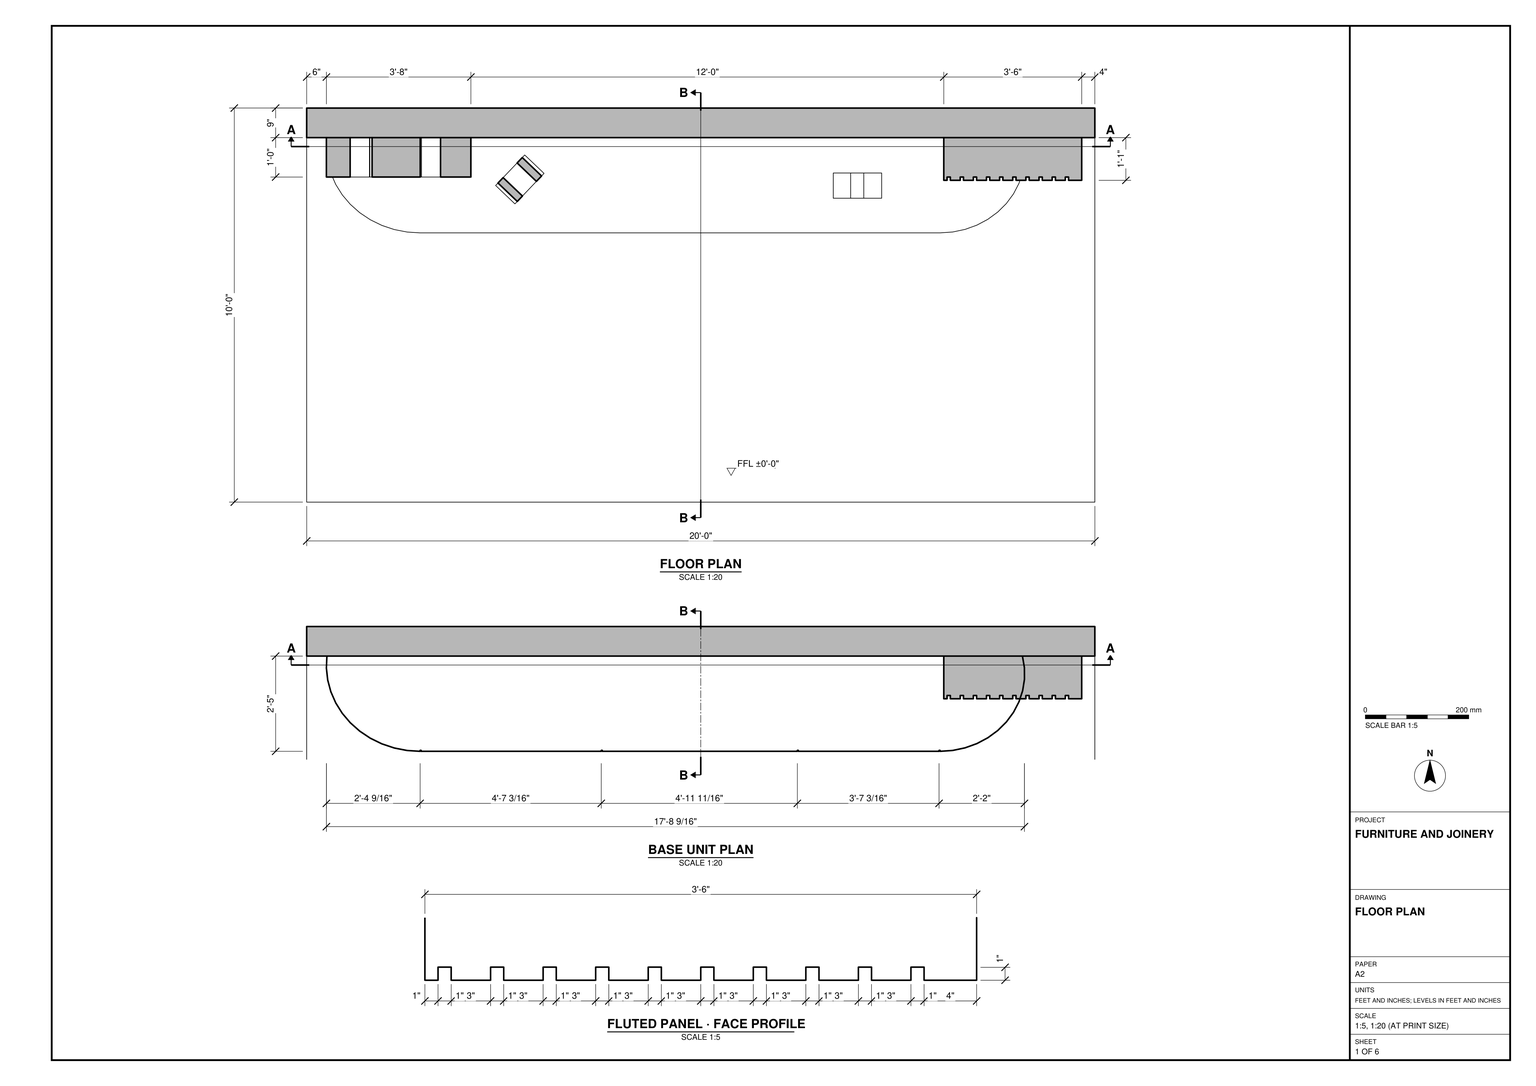
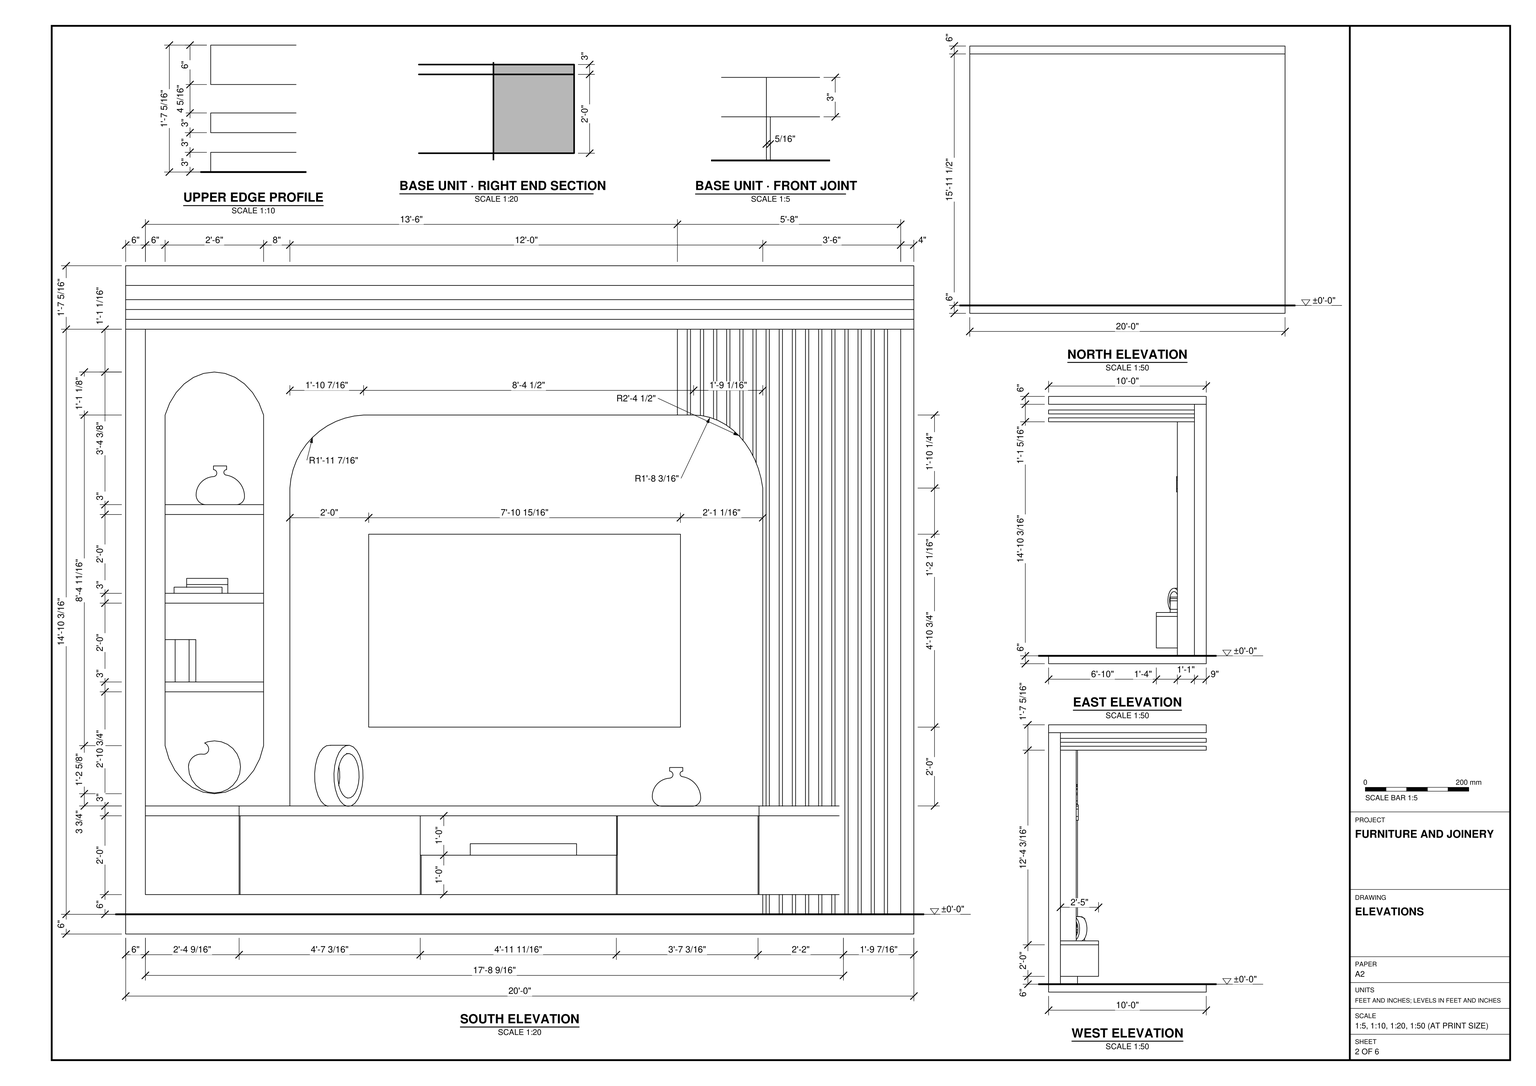
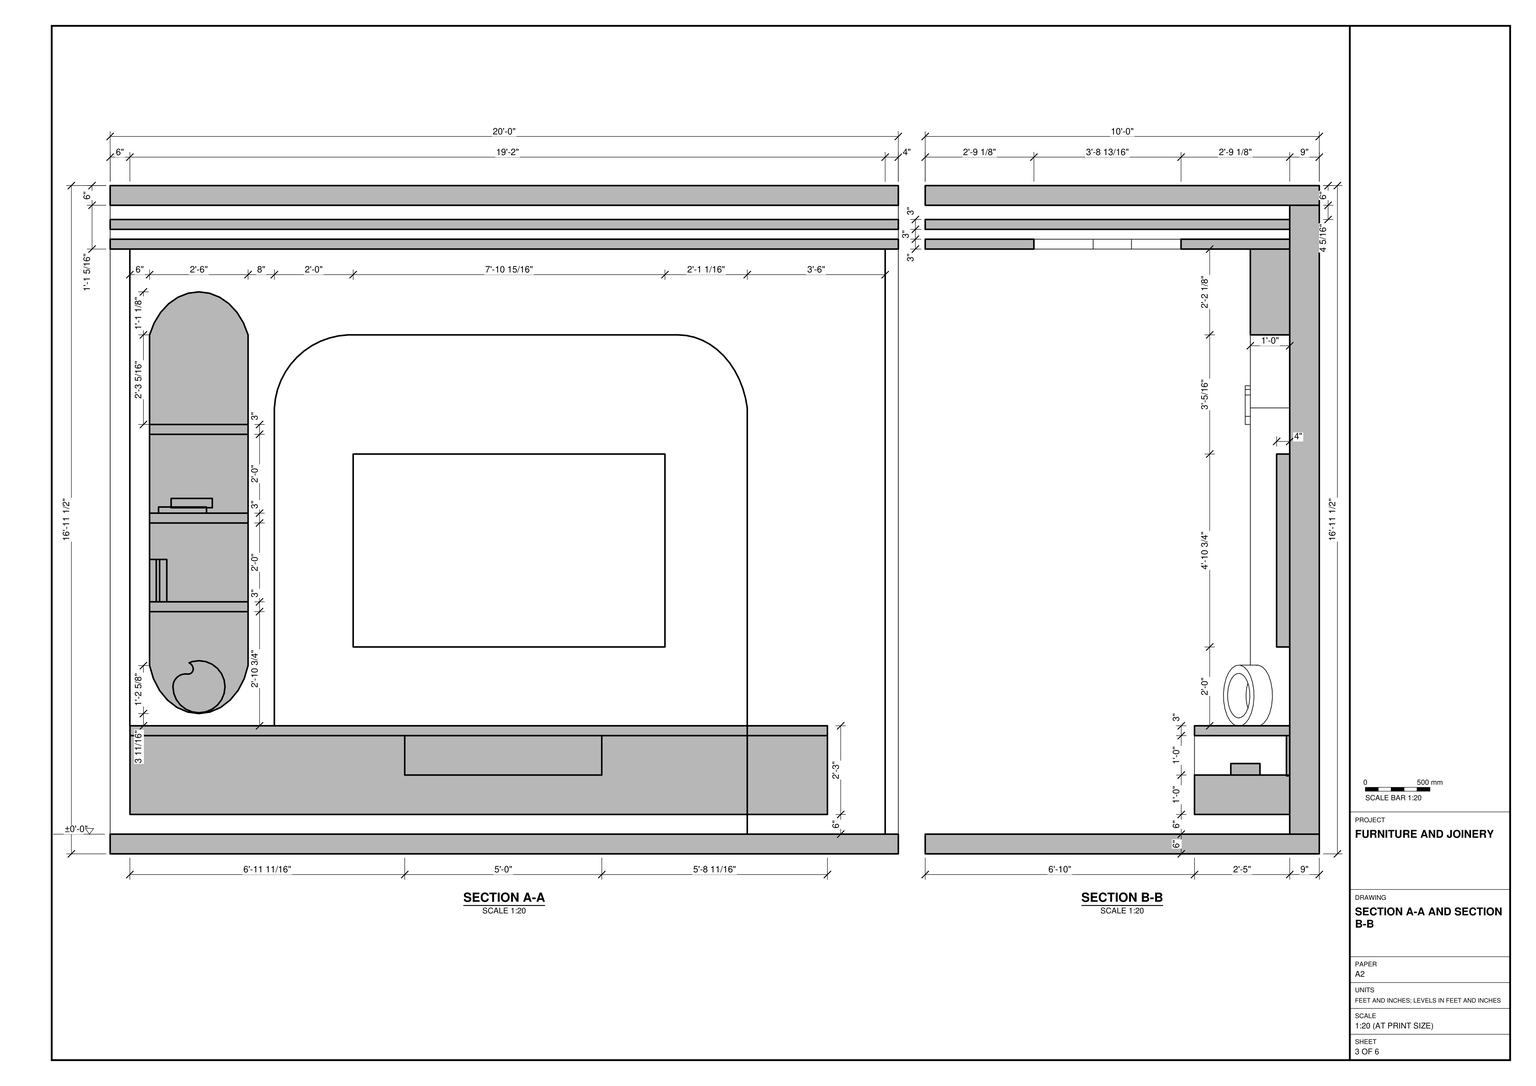
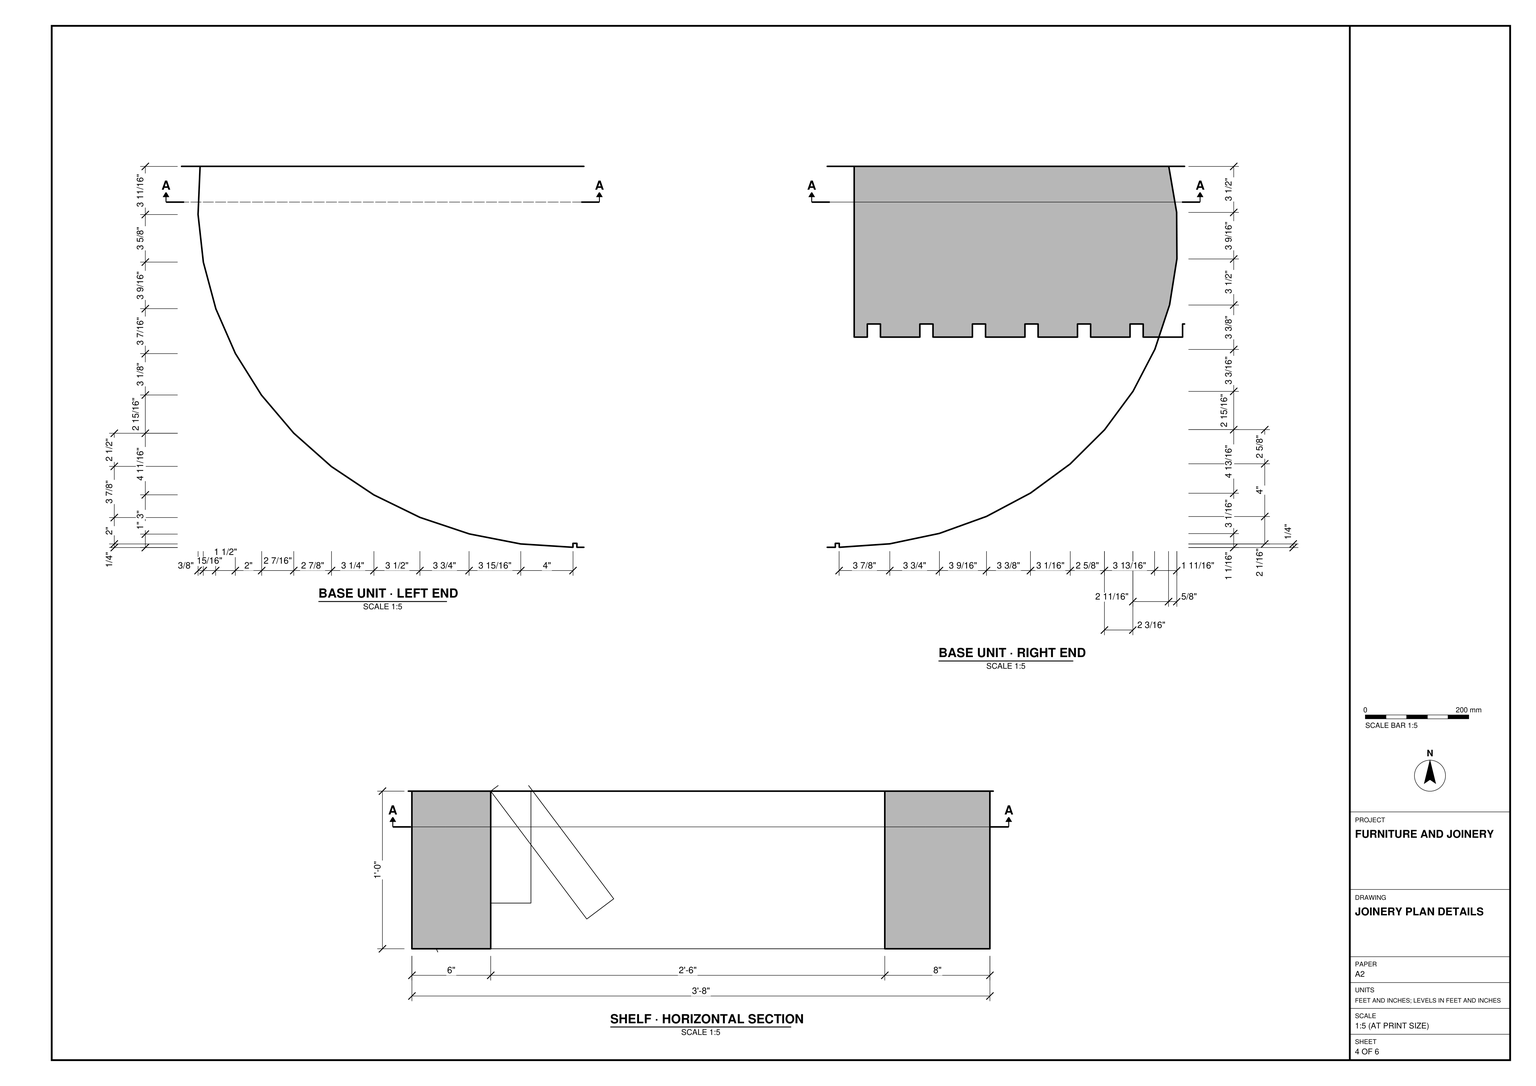
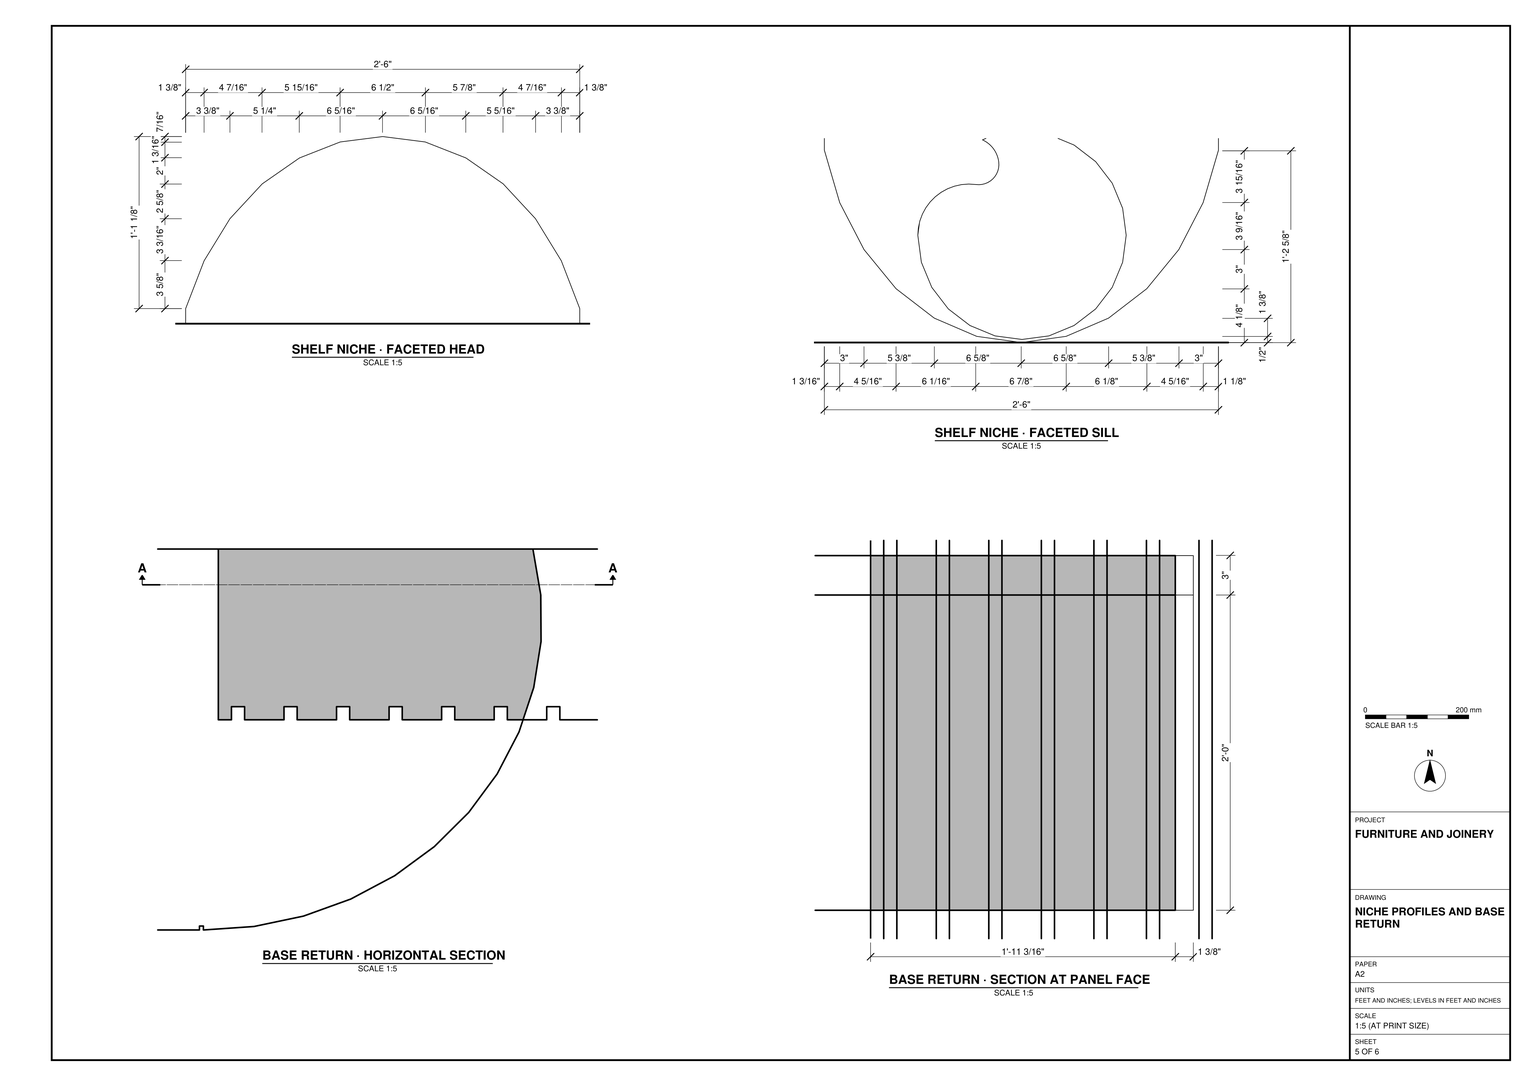
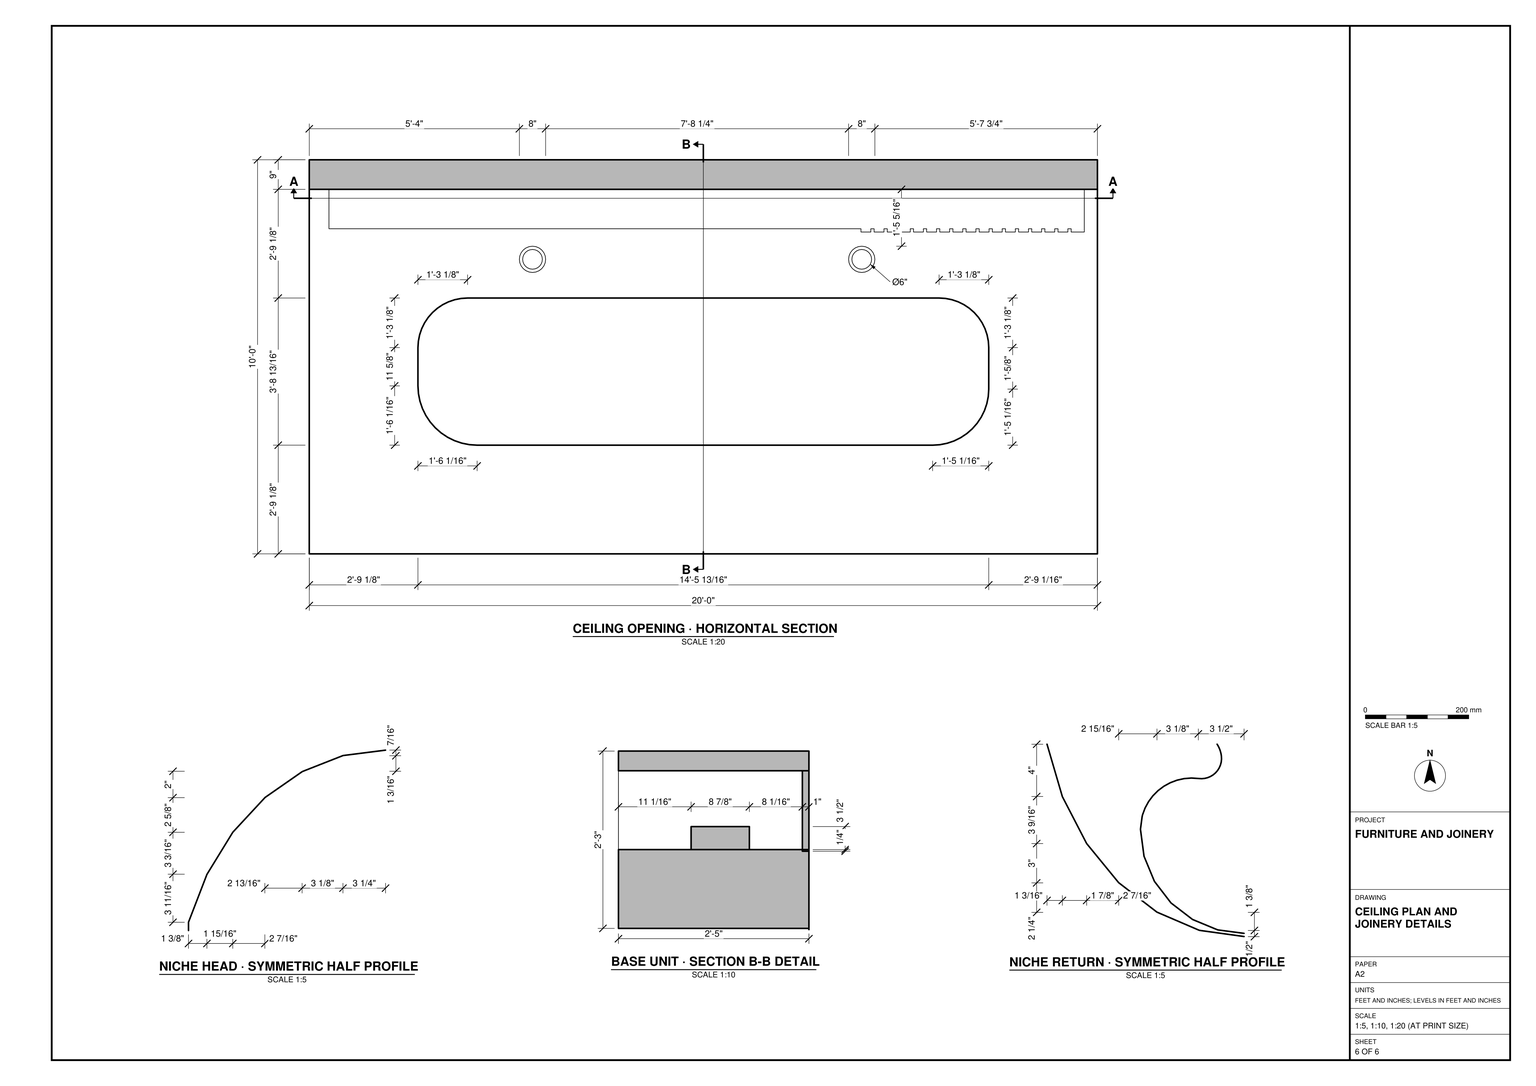
Build the TV wall and its surrounding floor, backing wall and overhead assembly in SketchUp from task_files/diagram_01.pdf. Work in feet and inches. The overall model is 20'-0" wide, 10'-0" deep and 16'-11 1/2" high. Set the finished floor at ±0'-0". Place the 9" backing wall along the north edge of the floor slab and use the south elevation to lay out the joinery.

Run the floating base cabinet beneath the shelving and TV. Follow the base unit plan for the straight front and curved ends, and the sections for the top thickness, divided fronts and open central compartment. Above the cabinet, form a tall, narrow display niche on the left with rounded upper and lower ends and horizontal shelves. Mount the rectangular TV within the wider central recess, keeping the straight head and rounded upper corners of the recess distinct from the TV itself. Model the vertical grooves in the right-hand panel and the stepped horizontal bands beneath the top slab.

Decor and loose items on the shelves and cabinet top may be any suitable library components placed as shown. Keep the shell elements and each joinery or furniture piece in separate groups or components, and use components for repeated parts. Save one SketchUp model as output_files/tv_wall_with_display_shelves_and_floating_storage.skp.

# SketchUp Ruby script. Lengths in inches.
U = 1.inch
M = Sketchup.active_model
def pt(a) = Geom::Point3d.new(a.map { |v| v * U })
def face(e, loops, mat)
  f = e.add_face(loops[0].map { |a| pt(a) })
  loops[1..].each { |l| e.add_face(l.map { |a| pt(a) }).erase! }
  f.material = f.back_material = mat if mat
  f
end
# faces: each face lists its corners as indices into pts; further lists are holes
def faces(e, pts, list, mat = nil) = list.each { |f| face(e, (f[0].is_a?(Array) ? f : [f]).map { |l| l.map { |i| pts[i] } }, mat) }
# xy, xz, yz: faces in a plane at the given z, y or x. An outline is a flat list of corners, or four numbers for a rectangle; further outlines are holes
def ring(l) = l.size == 4 ? [[l[0], l[1]], [l[2], l[1]], [l[2], l[3]], [l[0], l[3]]] : l.each_slice(2).to_a
def flat(e, list, mat, &to3) = list.each { |f| face(e, (f[0].is_a?(Array) ? f : [f]).map { |l| ring(l).map { |u, v| to3.(u, v) } }, mat) }
def xy(e, z, list, mat = nil) = flat(e, list, mat) { |x, y| [x, y, z] }
def xz(e, y, list, mat = nil) = flat(e, list, mat) { |x, z| [x, y, z] }
def yz(e, x, list, mat = nil) = flat(e, list, mat) { |y, z| [x, y, z] }
def lines(e, pts, list) = list.each { |a, b| e.add_line(pt(pts[a]), pt(pts[b])) }
# prism: a flat outline (further loops are holes) pulled along v
def prism(e, loops, v, mat = nil)
  f = face(e, loops, mat); d = Geom::Vector3d.new(v.map { |x| x * U })
  f.pushpull(f.normal.samedirection?(d) ? d.length : -d.length)
end
def box(e, o, s, mat = nil) = prism(e, [[o, [o[0] + s[0], o[1], o[2]], [o[0] + s[0], o[1] + s[1], o[2]], [o[0], o[1] + s[1], o[2]]]], [0, 0, s[2]], mat)
def at(x, y, z, deg = 0) = Geom::Transformation.translation(pt([x, y, z])) * Geom::Transformation.rotation(ORIGIN, Z_AXIS, deg.degrees)
def axes(o, x, y, z) = Geom::Transformation.new([*x, 0, *y, 0, *z, 0, *pt(o).to_a, 1])
def part(name) = M.definitions.add(name)
# library, detail: a bought-in or finely detailed component or shape, given as its bounding box
def library(name, o, s) = part(name).tap { |d| box(d.entities, o, s) }
def detail(e, o, s) = box(e.add_group.entities, o, s)
def put(e, d, t, mat = nil) = e.add_instance(d, t).tap { |i| i.material = mat if mat }
def group(e, t, mat = nil) = e.add_group.tap { |g| g.transformation = t; g.material = mat if mat }.entities
root = M.entities
M.materials.add("[Color A07]").color = [153, 0, 0]
M.materials.add("[Color E05]").color = [255, 255, 0]
M.materials.add("[Color E08]").color = [102, 102, 0]
M.materials.add("[Color L16]").color = [102, 0, 51]
M.materials.add("[Color M00]").color = [255, 255, 255]
M.materials.add("[Color M05]").color = [114, 114, 114]
M.materials.add("[Color M06]").color = [86, 86, 86]
M.materials.add("[Color M07]").color = [58, 58, 58]
M.materials.add("[Color M08]").color = [30, 30, 30]
M.materials.add("[Color M09]").color = [0, 0, 0]
c1 = part("Group\#17")
detail(c1.entities,[0,0,0],[14.74,7.6875,11.79])
g1 = group(root,at(0,0,0))
box(g1,[0,0,0],[240,120,6])
g2 = group(root,at(0,111,6),"[Color M00]")
box(g2,[0,0,0],[240,9,191.5])
g3 = group(root,at(6,99,39),"[Color M00]")
xy(g3,-33,[[188,-1,188,12,230,12,230,-1,226,-1,226,0,225,0,225,-1,222,-1,222,0,221,0,221,-1,218,-1,218,0,217,0,217,-1,214,-1,214,0,213,0,213,-1,210,-1,210,0,209,0,209,-1,206,-1,206,0,205,0,205,-1,202,-1,202,0,201,0,201,-1,198,-1,198,0,197,0,197,-1,194,-1,194,0,193,0,193,-1,190,-1,190,0,189,0,189,-1]])
xy(g3,0,[[0,0,44,12]])
xy(g3,119.04,[[162,-1,162,0,66.45,0,66.45,12,166.95,12,166.95,-1,166,-1,166,0,165,0,165,-1]])
xy(g3,145.17,[[162,-1,165,-1,165,0,166,0,166,-1,169,-1,169,0,170,0,170,-1,173,-1,173,0,174,0,174,-1,177,-1,177,0,178,0,178,-1,181,-1,181,0,182,0,182,-1,185,-1,185,0,186,0,186,-1,189,-1,189,0,190,0,190,-1,193,-1,193,0,194,0,194,-1,197,-1,197,0,198,0,198,-1,201,-1,201,0,202,0,202,-1,205,-1,205,0,206,0,206,-1,209,-1,209,0,210,0,210,-1,213,-1,213,0,214,0,214,-1,217,-1,217,0,218,0,218,-1,221,-1,221,0,222,0,222,-1,225,-1,225,0,226,0,226,-1,230,-1,230,12,0,12,0,0,162,0]])
xz(g3,-1,[[188,-33,189,-33,189,145.17,186,145.17,186,104.375,186.63,102.77,187.46,99.83,188,96.8],[190,-33,193,145.17],[194,-33,197,145.17],[198,-33,201,145.17],[202,-33,205,145.17],
  [206,-33,209,145.17],[210,-33,213,145.17],[214,-33,217,145.17],[218,-33,221,145.17],[222,-33,225,145.17],
  [226,-33,230,145.17],[185,106.59,185,145.17,182,145.17,182,111.27,182.59,110.57,184.18,108.17],[181,112.46,181,145.17,178,145.17,178,115.16,178.78,114.6,180.78,112.73],[177,115.89,177,145.17,174,145.17,174,117.53,174.32,117.41,176.61,116.17],[173,117.91,173,145.17,170,145.17,170,118.74,171.92,118.3125],
  [169,118.89,169,145.17,166,145.17,166,119.04,166.95,119.04],[162,119.04,165,145.17]],"[Color M08]")
xz(g3,0,[[[0,0,44,0,44,96.8,44.32,99.67,45,102.47,46.01,105.18,47.35,107.74,48.99,110.11,50.92,112.27,53.09,114.17,55.48,115.79,58.05,117.1,60.76,118.09,63.58,118.74,66.45,119.04,162,119.04,162,145.17,0,145.17],[21,3.73,17.6,4.2,14.36,5.59,11.46,7.83,9.02,10.81,7.17,14.38,6,18.37,6,119.04,7.4,122.68,9.37,125.89,11.83,128.53,14.66,130.51,17.76,131.73,21,132.14,24.24,131.73,27.34,130.51,30.17,128.53,32.63,125.89,34.6,122.68,36,119.04,36,18.37,34.83,14.38,32.98,10.81,30.54,7.83,27.64,5.59,24.4,4.2]]])
xz(g3,0,[[189,-33,190,145.17],[193,-33,194,145.17],[197,-33,198,145.17],[201,-33,202,145.17],[205,-33,206,145.17],
  [209,-33,210,145.17],[213,-33,214,145.17],[217,-33,218,145.17],[221,-33,222,145.17],[225,-33,226,145.17],
  [186,104.375,186,145.17,185,145.17,185,106.59,185.53,105.56],[182,111.27,182,145.17,181,145.17,181,112.46],[178,115.16,178,145.17,177,145.17,177,115.89],[174,117.53,174,145.17,173,145.17,173,117.91],[170,118.74,170,145.17,169,145.17,169,118.89,169.45,118.86],
  [165,119.04,166,145.17]],"[Color M08]")
xz(g3,12,[[[188,-33,188,96.8,187.46,99.83,186.63,102.77,185.53,105.56,184.18,108.17,182.59,110.57,180.78,112.73,178.78,114.6,176.61,116.17,174.32,117.41,171.92,118.3125,169.45,118.86,166.95,119.04,66.45,119.04,63.58,118.74,60.76,118.09,58.05,117.1,55.48,115.79,53.09,114.17,50.92,112.27,48.99,110.11,47.35,107.74,46.01,105.18,45,102.47,44.32,99.67,44,96.8,44,0,0,0,0,145.17,230,145.17,230,-33],[21,3.73,24.4,4.2,27.64,5.59,30.54,7.83,32.98,10.81,34.83,14.38,36,18.37,36,119.04,34.6,122.68,32.63,125.89,30.17,128.53,27.34,130.51,24.24,131.73,21,132.14,17.76,131.73,14.66,130.51,11.83,128.53,9.37,125.89,7.4,122.68,6,119.04,6,18.37,7.17,14.38,9.02,10.81,11.46,7.83,14.36,5.59,17.6,4.2]]])
yz(g3,0,[[0,0,12,145.17]])
yz(g3,6,[[0,18.37,12,119.04]])
yz(g3,36,[[0,18.37,12,119.04]])
yz(g3,44,[[0,0,12,96.8]])
yz(g3,162,[[-1,119.04,0,145.17]])
yz(g3,165,[[-1,119.04,0,145.17]])
yz(g3,166,[[-1,119.04,0,145.17]])
yz(g3,169,[[-1,118.89,0,145.17]])
yz(g3,170,[[-1,118.74,0,145.17]])
yz(g3,173,[[-1,117.91,0,145.17]])
yz(g3,174,[[-1,117.53,0,145.17]])
yz(g3,177,[[-1,115.89,0,145.17]])
yz(g3,178,[[-1,115.16,0,145.17]])
yz(g3,181,[[-1,112.46,0,145.17]])
yz(g3,182,[[-1,111.27,0,145.17]])
yz(g3,185,[[-1,106.59,0,145.17]])
yz(g3,186,[[-1,104.375,0,145.17]])
yz(g3,188,[[-1,-33,12,96.8]])
yz(g3,189,[[-1,-33,0,145.17]])
yz(g3,190,[[-1,-33,0,145.17]])
yz(g3,193,[[-1,-33,0,145.17]])
yz(g3,194,[[-1,-33,0,145.17]])
yz(g3,197,[[-1,-33,0,145.17]])
yz(g3,198,[[-1,-33,0,145.17]])
yz(g3,201,[[-1,-33,0,145.17]])
yz(g3,202,[[-1,-33,0,145.17]])
yz(g3,205,[[-1,-33,0,145.17]])
yz(g3,206,[[-1,-33,0,145.17]])
yz(g3,209,[[-1,-33,0,145.17]])
yz(g3,210,[[-1,-33,0,145.17]])
yz(g3,213,[[-1,-33,0,145.17]])
yz(g3,214,[[-1,-33,0,145.17]])
yz(g3,217,[[-1,-33,0,145.17]])
yz(g3,218,[[-1,-33,0,145.17]])
yz(g3,221,[[-1,-33,0,145.17]])
yz(g3,222,[[-1,-33,0,145.17]])
yz(g3,225,[[-1,-33,0,145.17]])
yz(g3,226,[[-1,-33,0,145.17]])
yz(g3,230,[[-1,-33,12,145.17]])
p = [[21,12,3.73],[17.6,12,4.2],[17.6,0,4.2],[21,0,3.73],[24.4,12,4.2],[24.4,0,4.2],
  [14.36,12,5.59],[14.36,0,5.59],[27.64,12,5.59],[27.64,0,5.59],[11.46,12,7.83],[11.46,0,7.83],
  [30.54,12,7.83],[30.54,0,7.83],[9.02,12,10.81],[9.02,0,10.81],[32.98,12,10.81],[32.98,0,10.81],
  [7.17,12,14.38],[7.17,0,14.38],[34.83,12,14.38],[34.83,0,14.38],[6,12,18.37],[6,0,18.37],
  [36,12,18.37],[36,0,18.37],[187.46,12,99.83],[188,12,96.8],[188,-1,96.8],[187.46,-1,99.83],
  [44.32,0,99.67],[44,0,96.8],[44,12,96.8],[44.32,12,99.67],[45,0,102.47],[45,12,102.47],
  [186.63,12,102.77],[186.63,-1,102.77],[46.01,0,105.18],[46.01,12,105.18],[185.53,12,105.56],[186,-1,104.375],
  [186,0,104.375],[185.53,0,105.56],[47.35,0,107.74],[47.35,12,107.74],[184.18,12,108.17],[185,0,106.59],
  [185,-1,106.59],[184.18,-1,108.17],[48.99,0,110.11],[48.99,12,110.11],[182.59,12,110.57],[182.59,-1,110.57],
  [50.92,0,112.27],[50.92,12,112.27],[180.78,12,112.73],[182,-1,111.27],[182,0,111.27],[181,0,112.46],
  [181,-1,112.46],[180.78,-1,112.73],[53.09,0,114.17],[53.09,12,114.17],[178.78,12,114.6],[178.78,-1,114.6],
  [55.48,0,115.79],[55.48,12,115.79],[176.61,12,116.17],[178,-1,115.16],[178,0,115.16],[177,0,115.89],
  [177,-1,115.89],[176.61,-1,116.17],[58.05,0,117.1],[58.05,12,117.1],[174.32,12,117.41],[174.32,-1,117.41],
  [60.76,0,118.09],[60.76,12,118.09],[171.92,12,118.3125],[174,-1,117.53],[174,0,117.53],[173,0,117.91],
  [173,-1,117.91],[171.92,-1,118.3125],[63.58,0,118.74],[63.58,12,118.74],[169.45,12,118.86],[170,-1,118.74],
  [170,0,118.74],[169.45,0,118.86],[66.45,0,119.04],[66.45,12,119.04],[166.95,12,119.04],[169,0,118.89],
  [169,-1,118.89],[166.95,-1,119.04],[6,12,119.04],[7.4,12,122.68],[7.4,0,122.68],[6,0,119.04],
  [34.6,12,122.68],[36,12,119.04],[36,0,119.04],[34.6,0,122.68],[9.37,12,125.89],[9.37,0,125.89],
  [32.63,12,125.89],[32.63,0,125.89],[11.83,12,128.53],[11.83,0,128.53],[30.17,12,128.53],[30.17,0,128.53],
  [14.66,12,130.51],[14.66,0,130.51],[27.34,12,130.51],[27.34,0,130.51],[17.76,12,131.73],[17.76,0,131.73],
  [24.24,12,131.73],[24.24,0,131.73],[21,12,132.14],[21,0,132.14]]
faces(g3,p,[[0,1,2,3],[4,0,3,5],[1,6,7,2],[8,4,5,9],[6,10,11,7],[12,8,9,13],[10,14,15,11],[16,12,13,17],
  [14,18,19,15],[20,16,17,21],[18,22,23,19],[24,20,21,25],[26,27,28,29],[30,31,32,33],[34,30,33,35],[36,26,29,37],
  [38,34,35,39],[40,36,37,41,42,43],[44,38,39,45],[46,40,43,47,48,49],[50,44,45,51],[52,46,49,53],[54,50,51,55],[56,52,53,57,58,59,60,61],
  [62,54,55,63],[64,56,61,65],[66,62,63,67],[68,64,65,69,70,71,72,73],[74,66,67,75],[76,68,73,77],[78,74,75,79],[80,76,77,81,82,83,84,85],
  [86,78,79,87],[88,80,85,89,90,91],[92,86,87,93],[94,88,91,95,96,97],[98,99,100,101],[102,103,104,105],[99,106,107,100],[108,102,105,109],
  [106,110,111,107],[112,108,109,113],[110,114,115,111],[116,112,113,117],[114,118,119,115],[120,116,117,121],[118,122,123,119],[122,120,121,123]])
g4 = group(root,at(6,82,36),"[Color M08]")
prism(g4,[[[0.16,29,0],[211.95,29,0],[212.55,25.5,0],[212.57,21.96,0],[212.01,18.46,0],[210.89,15.07,0],[209.23,11.875,0],[207.06,8.94,0],[204.4375,6.34,0],[201.42,4.13,0],[198.08,2.35,0],[194.48,1.06,0],[190.72,0.27,0],[186.86,0,0],[28.54,0,0],[24.56,0.26,0],[20.65,1.02,0],[16.9,2.27,0],[13.375,3.99,0],[10.15,6.15,0],[7.28,8.7,0],[4.83,11.58,0],[2.84,14.76,0],[1.36,18.15,0],[0.4,21.7,0],[0,25.34,0]]],[0,0,3])
g5 = group(root,at(6,82,12),"[Color M00]")
xy(g5,0,[[28.54,0,24.56,0.26,20.65,1.02,16.9,2.27,13.375,3.99,10.15,6.15,7.28,8.7,4.83,11.58,2.84,14.76,1.36,18.15,0.4,21.7,0,25.34,0.16,29,211.95,29,212.55,25.5,212.57,21.96,212.01,18.46,210.89,15.07,209.23,11.875,207.06,8.94,204.4375,6.34,201.42,4.13,198.08,2.35,194.48,1.06,190.72,0.27,186.86,0,186.86,0.3,186.5625,0.3,186.5625,0,143.7,0,143.7,0.3,143.4,0.3,143.4,0,84,0,84,0.3,83.7,0.3,83.7,0,28.84,0,28.84,0.3,28.54,0.3]])
xy(g5,12,[[84,0,143.4,0,143.4,0.3,143.7,0.3,143.7,29,83.7,29,83.7,0.3,84,0.3]],"[Color M09]")
xy(g5,24,[[28.54,0,28.54,0.3,28.84,0.3,28.84,0,83.7,0,83.7,29,0.16,29,0,25.34,0.4,21.7,1.36,18.15,2.84,14.76,4.83,11.58,7.28,8.7,10.15,6.15,13.375,3.99,16.9,2.27,20.65,1.02,24.56,0.26],[143.7,0,186.5625,0,186.5625,0.3,186.86,0.3,186.86,0,190.72,0.27,194.48,1.06,198.08,2.35,201.42,4.13,204.4375,6.34,207.06,8.94,209.23,11.875,210.89,15.07,212.01,18.46,212.57,21.96,212.55,25.5,211.95,29,143.7,29]])
xz(g5,0,[[28.84,0,83.7,24],[84,0,143.4,12],[143.7,0,186.5625,24]])
xz(g5,0.3,[[28.54,0,28.84,24],[83.7,0,84,12],[143.4,0,143.7,12],[186.5625,0,186.86,24]])
xz(g5,29,[[0.16,0,0.16,24,83.7,24,83.7,12,143.7,12,143.7,24,211.95,24,211.95,0]])
yz(g5,28.54,[[0,0,0.3,24]])
yz(g5,28.84,[[0,0,0.3,24]])
yz(g5,83.7,[[0,0,0.3,12]])
yz(g5,83.7,[[0,12,29,24]],"[Color M09]")
yz(g5,84,[[0,0,0.3,12]])
yz(g5,143.4,[[0,0,0.3,12]])
yz(g5,143.7,[[0,0,0.3,12]])
yz(g5,143.7,[[0,12,29,24]],"[Color M09]")
yz(g5,186.5625,[[0,0,0.3,24]])
yz(g5,186.86,[[0,0,0.3,24]])
p = [[28.54,0,24],[24.56,0.26,24],[24.56,0.26,0],[28.54,0,0],[190.72,0.27,24],[186.86,0,24],
  [186.86,0,0],[190.72,0.27,0],[20.65,1.02,24],[20.65,1.02,0],[194.48,1.06,24],[194.48,1.06,0],
  [16.9,2.27,24],[16.9,2.27,0],[198.08,2.35,24],[198.08,2.35,0],[13.375,3.99,24],[13.375,3.99,0],
  [201.42,4.13,24],[201.42,4.13,0],[10.15,6.15,24],[10.15,6.15,0],[204.4375,6.34,24],[204.4375,6.34,0],
  [7.28,8.7,24],[7.28,8.7,0],[207.06,8.94,24],[207.06,8.94,0],[4.83,11.58,24],[4.83,11.58,0],
  [209.23,11.875,24],[209.23,11.875,0],[2.84,14.76,24],[2.84,14.76,0],[210.89,15.07,24],[210.89,15.07,0],
  [1.36,18.15,24],[1.36,18.15,0],[212.01,18.46,24],[212.01,18.46,0],[0.4,21.7,24],[0.4,21.7,0],
  [212.57,21.96,24],[212.57,21.96,0],[0,25.34,24],[0,25.34,0],[212.55,25.5,24],[212.55,25.5,0],
  [0.16,29,24],[0.16,29,0],[211.95,29,24],[211.95,29,0]]
faces(g5,p,[[0,1,2,3],[4,5,6,7],[1,8,9,2],[10,4,7,11],[8,12,13,9],[14,10,11,15],[12,16,17,13],[18,14,15,19],
  [16,20,21,17],[22,18,19,23],[20,24,25,21],[26,22,23,27],[24,28,29,25],[30,26,27,31],[28,32,33,29],[34,30,31,35],
  [32,36,37,33],[38,34,35,39],[36,40,41,37],[42,38,39,43],[40,44,45,41],[46,42,43,47],[44,48,49,45],[50,46,47,51]])
g6 = group(root,at(12,99,127.75),"[Color M06]")
box(g6,[0,0,0],[30,12,3])
g7 = group(root,at(12,99,100.75),"[Color M06]")
box(g7,[0,0,0],[30,12,3])
g8 = group(root,at(12,99,73.75),"[Color M06]")
box(g8,[0,0,0],[30,12,3])
g9 = group(root,at(74,107,63),"[Color M09]")
box(g9,[0,0,0],[94.9375,4,58.75])
g10 = group(root,at(0,0,184.17),"[Color M00]")
xy(g10,0,[[[0,0,240,111],[51.14,33.09,189.83,33.09,192.05,33.24,194.25,33.68,196.36,34.39,198.37,35.38,200.22,36.625,201.9,38.1,203.375,39.78,204.62,41.63,205.61,43.64,206.32,45.75,206.76,47.95,206.91,50.17,206.91,62.81,206.78,64.78,206.39,66.71,205.76,68.58,204.88,70.36,203.79,72,202.48,73.48,201,74.79,199.36,75.88,197.58,76.76,195.71,77.39,193.78,77.78,191.81,77.91,48.2,77.91,46.22,77.78,44.29,77.39,42.42,76.76,40.64,75.88,39,74.78,37.52,73.48,36.22,72,35.12,70.36,34.24,68.58,33.61,66.71,33.22,64.78,33.09,62.8,33.09,51.14,33.25,48.79,33.71,46.47,34.47,44.23,35.51,42.12,36.82,40.15,38.38,38.38,40.15,36.82,42.12,35.51,44.23,34.47,46.47,33.71,48.79,33.25],[67.98,85.6875,69.01,85.82,69.98,86.22,70.81,86.86,71.44,87.6875,71.84,88.65,71.98,89.6875,71.84,90.72,71.44,91.6875,70.81,92.52,69.98,93.15,69.01,93.55,67.98,93.6875,66.94,93.55,65.98,93.15,65.15,92.52,64.51,91.6875,64.11,90.72,63.98,89.6875,64.11,88.65,64.51,87.6875,65.15,86.86,65.98,86.22,66.94,85.82],[168.23,85.6875,169.26,85.82,170.23,86.22,171.06,86.86,171.69,87.6875,172.09,88.65,172.23,89.6875,172.09,90.72,171.69,91.6875,171.06,92.52,170.23,93.15,169.26,93.55,168.23,93.6875,167.19,93.55,166.23,93.15,165.4,92.52,164.76,91.6875,164.36,90.72,164.23,89.6875,164.36,88.65,164.76,87.6875,165.4,86.86,166.23,86.22,167.19,85.82]]])
xy(g10,0.3125,[[[168.23,85.6875,167.19,85.82,166.23,86.22,165.4,86.86,164.76,87.6875,164.36,88.65,164.23,89.6875,164.36,90.72,164.76,91.6875,165.4,92.52,166.23,93.15,167.19,93.55,168.23,93.6875,169.26,93.55,170.23,93.15,171.06,92.52,171.69,91.6875,172.09,90.72,172.23,89.6875,172.09,88.65,171.69,87.6875,171.06,86.86,170.23,86.22,169.26,85.82],[168.23,86.6875,169,86.79,169.73,87.09,170.35,87.57,170.83,88.1875,171.125,88.91,171.23,89.6875,171.125,90.46,170.83,91.1875,170.35,91.81,169.73,92.29,169,92.59,168.23,92.6875,167.45,92.59,166.73,92.29,166.11,91.81,165.63,91.1875,165.33,90.46,165.23,89.6875,165.33,88.91,165.63,88.1875,166.11,87.57,166.73,87.09,167.45,86.79]]],"[Color M00]")
xy(g10,0.6,[[[67.98,85.6875,66.94,85.82,65.98,86.22,65.15,86.86,64.51,87.6875,64.11,88.65,63.98,89.6875,64.11,90.72,64.51,91.6875,65.15,92.52,65.98,93.15,66.94,93.55,67.98,93.6875,69.01,93.55,69.98,93.15,70.81,92.52,71.44,91.6875,71.84,90.72,71.98,89.6875,71.84,88.65,71.44,87.6875,70.81,86.86,69.98,86.22,69.01,85.82],[67.98,86.6875,68.75,86.79,69.48,87.09,70.1,87.57,70.58,88.1875,70.875,88.91,70.98,89.6875,70.875,90.46,70.58,91.1875,70.1,91.81,69.48,92.29,68.75,92.59,67.98,92.6875,67.2,92.59,66.48,92.29,65.86,91.81,65.38,91.1875,65.08,90.46,64.98,89.6875,65.08,88.91,65.38,88.1875,65.86,87.57,66.48,87.09,67.2,86.79]]],"[Color M00]")
xy(g10,1,[[67.98,86.6875,67.2,86.79,66.48,87.09,65.86,87.57,65.38,88.1875,65.08,88.91,64.98,89.6875,65.08,90.46,65.38,91.1875,65.86,91.81,66.48,92.29,67.2,92.59,67.98,92.6875,68.75,92.59,69.48,92.29,70.1,91.81,70.58,91.1875,70.875,90.46,70.98,89.6875,70.875,88.91,70.58,88.1875,70.1,87.57,69.48,87.09,68.75,86.79]],"[Color M00]")
xy(g10,1.125,[[168.23,86.6875,167.45,86.79,166.73,87.09,166.11,87.57,165.63,88.1875,165.33,88.91,165.23,89.6875,165.33,90.46,165.63,91.1875,166.11,91.81,166.73,92.29,167.45,92.59,168.23,92.6875,169,92.59,169.73,92.29,170.35,91.81,170.83,91.1875,171.125,90.46,171.23,89.6875,171.125,88.91,170.83,88.1875,170.35,87.57,169.73,87.09,169,86.79]],"[Color M00]")
xy(g10,3,[[[0,0,240,111],[51.14,33.09,48.79,33.25,46.47,33.71,44.23,34.47,42.12,35.51,40.15,36.82,38.38,38.38,36.82,40.15,35.51,42.12,34.47,44.23,33.71,46.47,33.25,48.79,33.09,51.14,33.09,62.8,33.22,64.78,33.61,66.71,34.24,68.58,35.12,70.36,36.22,72,37.52,73.48,39,74.78,40.64,75.88,42.42,76.76,44.29,77.39,46.22,77.78,48.2,77.91,191.81,77.91,193.78,77.78,195.71,77.39,197.58,76.76,199.36,75.88,201,74.79,202.48,73.48,203.79,72,204.88,70.36,205.76,68.58,206.39,66.71,206.78,64.78,206.91,62.81,206.91,50.17,206.76,47.95,206.32,45.75,205.61,43.64,204.62,41.63,203.375,39.78,201.9,38.1,200.22,36.625,198.37,35.38,196.36,34.39,194.25,33.68,192.05,33.24,189.83,33.09]]])
xz(g10,0,[[0,0,240,3]])
xz(g10,33.09,[[51.14,0,189.83,3]])
xz(g10,77.91,[[48.2,0,191.81,3]])
xz(g10,111,[[0,0,240,3]])
yz(g10,0,[[0,0,111,3]])
yz(g10,33.09,[[51.14,0,62.8,3]])
yz(g10,206.91,[[50.17,0,62.81,3]])
yz(g10,240,[[0,0,111,3]])
p = [[51.14,33.09,0],[48.79,33.25,0],[48.79,33.25,3],[51.14,33.09,3],[192.05,33.24,0],[189.83,33.09,0],
  [189.83,33.09,3],[192.05,33.24,3],[46.47,33.71,0],[46.47,33.71,3],[194.25,33.68,0],[194.25,33.68,3],
  [44.23,34.47,0],[44.23,34.47,3],[196.36,34.39,0],[196.36,34.39,3],[198.37,35.38,0],[198.37,35.38,3],
  [42.12,35.51,0],[42.12,35.51,3],[200.22,36.625,0],[200.22,36.625,3],[40.15,36.82,0],[40.15,36.82,3],
  [201.9,38.1,0],[201.9,38.1,3],[38.38,38.38,0],[38.38,38.38,3],[203.375,39.78,0],[203.375,39.78,3],
  [36.82,40.15,0],[36.82,40.15,3],[204.62,41.63,0],[204.62,41.63,3],[35.51,42.12,0],[35.51,42.12,3],
  [205.61,43.64,0],[205.61,43.64,3],[34.47,44.23,0],[34.47,44.23,3],[206.32,45.75,0],[206.32,45.75,3],
  [33.71,46.47,0],[33.71,46.47,3],[206.76,47.95,0],[206.76,47.95,3],[33.25,48.79,0],[33.25,48.79,3],
  [206.91,50.17,0],[206.91,50.17,3],[33.09,51.14,0],[33.09,51.14,3],[33.09,62.8,0],[33.22,64.78,0],
  [33.22,64.78,3],[33.09,62.8,3],[206.78,64.78,0],[206.91,62.81,0],[206.91,62.81,3],[206.78,64.78,3],
  [33.61,66.71,0],[33.61,66.71,3],[206.39,66.71,0],[206.39,66.71,3],[34.24,68.58,0],[34.24,68.58,3],
  [205.76,68.58,0],[205.76,68.58,3],[35.12,70.36,0],[35.12,70.36,3],[204.88,70.36,0],[204.88,70.36,3],
  [36.22,72,0],[36.22,72,3],[203.79,72,0],[203.79,72,3],[37.52,73.48,0],[37.52,73.48,3],
  [202.48,73.48,0],[202.48,73.48,3],[39,74.78,0],[39,74.78,3],[201,74.79,0],[201,74.79,3],
  [40.64,75.88,0],[40.64,75.88,3],[199.36,75.88,0],[199.36,75.88,3],[42.42,76.76,0],[42.42,76.76,3],
  [197.58,76.76,0],[197.58,76.76,3],[44.29,77.39,0],[44.29,77.39,3],[195.71,77.39,0],[195.71,77.39,3],
  [46.22,77.78,0],[46.22,77.78,3],[193.78,77.78,0],[193.78,77.78,3],[48.2,77.91,0],[48.2,77.91,3],
  [191.81,77.91,0],[191.81,77.91,3],[67.98,85.6875,0],[66.94,85.82,0],[66.94,85.82,0.6],[67.98,85.6875,0.6],
  [69.01,85.82,0],[69.01,85.82,0.6],[168.23,85.6875,0],[167.19,85.82,0],[167.19,85.82,0.3125],[168.23,85.6875,0.3125],
  [169.26,85.82,0],[169.26,85.82,0.3125],[65.98,86.22,0],[65.98,86.22,0.6],[69.98,86.22,0],[69.98,86.22,0.6],
  [166.23,86.22,0],[166.23,86.22,0.3125],[170.23,86.22,0],[170.23,86.22,0.3125],[65.15,86.86,0],[65.15,86.86,0.6],
  [70.81,86.86,0],[70.81,86.86,0.6],[165.4,86.86,0],[165.4,86.86,0.3125],[171.06,86.86,0],[171.06,86.86,0.3125],
  [64.51,87.6875,0],[64.51,87.6875,0.6],[71.44,87.6875,0],[71.44,87.6875,0.6],[164.76,87.6875,0],[164.76,87.6875,0.3125],
  [171.69,87.6875,0],[171.69,87.6875,0.3125],[64.11,88.65,0],[64.11,88.65,0.6],[71.84,88.65,0],[71.84,88.65,0.6],
  [164.36,88.65,0],[164.36,88.65,0.3125],[172.09,88.65,0],[172.09,88.65,0.3125],[63.98,89.6875,0],[63.98,89.6875,0.6],
  [71.98,89.6875,0],[71.98,89.6875,0.6],[164.23,89.6875,0],[164.23,89.6875,0.3125],[172.23,89.6875,0],[172.23,89.6875,0.3125],
  [64.11,90.72,0],[64.11,90.72,0.6],[71.84,90.72,0],[71.84,90.72,0.6],[164.36,90.72,0],[164.36,90.72,0.3125],
  [172.09,90.72,0],[172.09,90.72,0.3125],[64.51,91.6875,0],[64.51,91.6875,0.6],[71.44,91.6875,0],[71.44,91.6875,0.6],
  [164.76,91.6875,0],[164.76,91.6875,0.3125],[171.69,91.6875,0],[171.69,91.6875,0.3125],[65.15,92.52,0],[65.15,92.52,0.6],
  [70.81,92.52,0],[70.81,92.52,0.6],[165.4,92.52,0],[165.4,92.52,0.3125],[171.06,92.52,0],[171.06,92.52,0.3125],
  [65.98,93.15,0],[65.98,93.15,0.6],[69.98,93.15,0],[69.98,93.15,0.6],[166.23,93.15,0],[166.23,93.15,0.3125],
  [170.23,93.15,0],[170.23,93.15,0.3125],[66.94,93.55,0],[66.94,93.55,0.6],[69.01,93.55,0],[69.01,93.55,0.6],
  [167.19,93.55,0],[167.19,93.55,0.3125],[169.26,93.55,0],[169.26,93.55,0.3125],[67.98,93.6875,0],[67.98,93.6875,0.6],
  [168.23,93.6875,0],[168.23,93.6875,0.3125],[168.23,86.6875,1.125],[168.23,86.6875,0.3125],[167.45,86.79,0.3125],[167.45,86.79,1.125],
  [169,86.79,1.125],[169,86.79,0.3125],[166.73,87.09,0.3125],[166.73,87.09,1.125],[169.73,87.09,1.125],[169.73,87.09,0.3125],
  [166.11,87.57,0.3125],[166.11,87.57,1.125],[170.35,87.57,1.125],[170.35,87.57,0.3125],[165.63,88.1875,0.3125],[165.63,88.1875,1.125],
  [170.83,88.1875,1.125],[170.83,88.1875,0.3125],[165.33,88.91,0.3125],[165.33,88.91,1.125],[171.125,88.91,1.125],[171.125,88.91,0.3125],
  [165.23,89.6875,0.3125],[165.23,89.6875,1.125],[171.23,89.6875,1.125],[171.23,89.6875,0.3125],[165.33,90.46,0.3125],[165.33,90.46,1.125],
  [171.125,90.46,1.125],[171.125,90.46,0.3125],[165.63,91.1875,0.3125],[165.63,91.1875,1.125],[170.83,91.1875,1.125],[170.83,91.1875,0.3125],
  [166.11,91.81,0.3125],[166.11,91.81,1.125],[170.35,91.81,1.125],[170.35,91.81,0.3125],[166.73,92.29,0.3125],[166.73,92.29,1.125],
  [169.73,92.29,1.125],[169.73,92.29,0.3125],[167.45,92.59,0.3125],[167.45,92.59,1.125],[169,92.59,1.125],[169,92.59,0.3125],
  [168.23,92.6875,0.3125],[168.23,92.6875,1.125],[67.98,86.6875,1],[67.98,86.6875,0.6],[67.2,86.79,0.6],[67.2,86.79,1],
  [68.75,86.79,1],[68.75,86.79,0.6],[66.48,87.09,0.6],[66.48,87.09,1],[69.48,87.09,1],[69.48,87.09,0.6],
  [65.86,87.57,0.6],[65.86,87.57,1],[70.1,87.57,1],[70.1,87.57,0.6],[65.38,88.1875,0.6],[65.38,88.1875,1],
  [70.58,88.1875,1],[70.58,88.1875,0.6],[65.08,88.91,0.6],[65.08,88.91,1],[70.875,88.91,1],[70.875,88.91,0.6],
  [64.98,89.6875,0.6],[64.98,89.6875,1],[70.98,89.6875,1],[70.98,89.6875,0.6],[65.08,90.46,0.6],[65.08,90.46,1],
  [70.875,90.46,1],[70.875,90.46,0.6],[65.38,91.1875,0.6],[65.38,91.1875,1],[70.58,91.1875,1],[70.58,91.1875,0.6],
  [65.86,91.81,0.6],[65.86,91.81,1],[70.1,91.81,1],[70.1,91.81,0.6],[66.48,92.29,0.6],[66.48,92.29,1],
  [69.48,92.29,1],[69.48,92.29,0.6],[67.2,92.59,0.6],[67.2,92.59,1],[68.75,92.59,1],[68.75,92.59,0.6],
  [67.98,92.6875,0.6],[67.98,92.6875,1]]
faces(g10,p,[[0,1,2,3],[4,5,6,7],[1,8,9,2],[10,4,7,11],[8,12,13,9],[14,10,11,15],[16,14,15,17],[12,18,19,13],
  [20,16,17,21],[18,22,23,19],[24,20,21,25],[22,26,27,23],[28,24,25,29],[26,30,31,27],[32,28,29,33],[30,34,35,31],
  [36,32,33,37],[34,38,39,35],[40,36,37,41],[38,42,43,39],[44,40,41,45],[42,46,47,43],[48,44,45,49],[46,50,51,47],
  [52,53,54,55],[56,57,58,59],[53,60,61,54],[62,56,59,63],[60,64,65,61],[66,62,63,67],[64,68,69,65],[70,66,67,71],
  [68,72,73,69],[74,70,71,75],[72,76,77,73],[78,74,75,79],[76,80,81,77],[82,78,79,83],[80,84,85,81],[86,82,83,87],
  [84,88,89,85],[90,86,87,91],[88,92,93,89],[94,90,91,95],[92,96,97,93],[98,94,95,99],[96,100,101,97],[102,98,99,103]])
faces(g10,p,[[104,105,106,107],[108,104,107,109],[110,111,112,113],[114,110,113,115],[105,116,117,106],[118,108,109,119],[111,120,121,112],[122,114,115,123],
  [116,124,125,117],[126,118,119,127],[120,128,129,121],[130,122,123,131],[124,132,133,125],[134,126,127,135],[128,136,137,129],[138,130,131,139],
  [132,140,141,133],[142,134,135,143],[136,144,145,137],[146,138,139,147],[140,148,149,141],[150,142,143,151],[144,152,153,145],[154,146,147,155],
  [148,156,157,149],[158,150,151,159],[152,160,161,153],[162,154,155,163],[156,164,165,157],[166,158,159,167],[160,168,169,161],[170,162,163,171],
  [164,172,173,165],[174,166,167,175],[168,176,177,169],[178,170,171,179],[172,180,181,173],[182,174,175,183],[176,184,185,177],[186,178,179,187],
  [180,188,189,181],[190,182,183,191],[184,192,193,185],[194,186,187,195],[188,196,197,189],[196,190,191,197],[192,198,199,193],[198,194,195,199],
  [200,201,202,203],[204,205,201,200],[203,202,206,207],[208,209,205,204],[207,206,210,211],[212,213,209,208],[211,210,214,215],[216,217,213,212],
  [215,214,218,219],[220,221,217,216],[219,218,222,223],[224,225,221,220],[223,222,226,227],[228,229,225,224],[227,226,230,231],[232,233,229,228],
  [231,230,234,235],[236,237,233,232],[235,234,238,239],[240,241,237,236],[239,238,242,243],[244,245,241,240],[243,242,246,247],[247,246,245,244],
  [248,249,250,251],[252,253,249,248],[251,250,254,255],[256,257,253,252],[255,254,258,259],[260,261,257,256],[259,258,262,263],[264,265,261,260],
  [263,262,266,267],[268,269,265,264],[267,266,270,271],[272,273,269,268],[271,270,274,275],[276,277,273,272],[275,274,278,279],[280,281,277,276],
  [279,278,282,283],[284,285,281,280],[283,282,286,287],[288,289,285,284],[287,286,290,291],[292,293,289,288],[291,290,294,295],[295,294,293,292]],"[Color M00]")
g11 = group(root,at(0,0,190.17),"[Color M00]")
box(g11,[0,0,0],[240,111,3])
g12 = group(root,at(0,0,197.5))
box(g12,[0,0,0],[240,120,6])
g13 = group(root,at(89.7,110,23.75),"[Color M09]")
box(g13,[0,0,0],[59.8125,1,12.25])
g14 = group(root,at(12,101.27,76.75),"[Color L16]")
xy(g14,0,[[7.3125,0,3.0625,5.66,3.0625,9.73,0,9.73,2.05,11.27,9.36,1.54],[0,1.21,0,9.73,3.0625,5.66,3.0625,1.21],[3.0625,5.66,0,9.73,3.0625,9.73]])
xy(g14,12.9,[[7.3125,0,9.36,1.54,2.05,11.27,0,9.73,3.0625,9.73,3.0625,5.66],[0,1.21,3.0625,1.21,3.0625,5.66,0,9.73],[3.0625,5.66,3.0625,9.73,0,9.73]])
xz(g14,1.21,[[0,0,3.0625,12.9]])
xz(g14,9.73,[[0,0,3.0625,12.9]])
yz(g14,0,[[1.21,0,9.73,12.9]])
yz(g14,3.0625,[[1.21,0,9.73,12.9]])
p = [[7.3125,0,0],[7.3125,0,12.9],[3.0625,5.66,12.9],[0,9.73,12.9],[0,9.73,0],[3.0625,5.66,0],
  [9.36,1.54,0],[9.36,1.54,12.9],[2.05,11.27,0],[2.05,11.27,12.9]]
faces(g14,p,[[0,1,2,3,4,5],[1,0,6,7],[7,6,8,9],[4,3,9,8]])
g15 = group(root,at(14.74,99,103.75),"[Color A07]")
box(g15,[0,0,0],[14.61,10.18,1.875])
g16 = group(root,at(18.57,100.84,103.75),"[Color A07]")
prism(g16,[[[12.54,0.65,0],[12.54,8.34,1.875],[12.54,7.6875,4.55],[12.54,0,2.67]]],[-12.54,0,0])
put(root,c1,at(21.45,97.4375,130.75),"[Color M09]")
g17 = group(root,at(63.42,90.82,38.88),"[Color M07]")
detail(g17,[-5.88,0,0],[14.74,14.9,18.59])
g18 = group(root,at(19.11,99,42.96),"[Color E05]")
detail(g18,[0,0,0],[15.86,12,15.86])
put(root,c1,at(160.35,92.54,38.92),"[Color E08]")
g19 = group(root,at(104.93,93.06,24),"[Color M05]")
box(g19,[0,0,0],[32.375,8.875,3.5])
